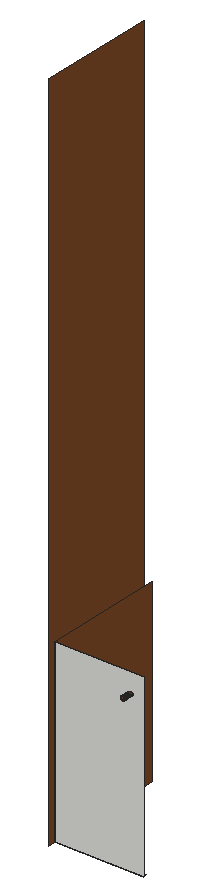
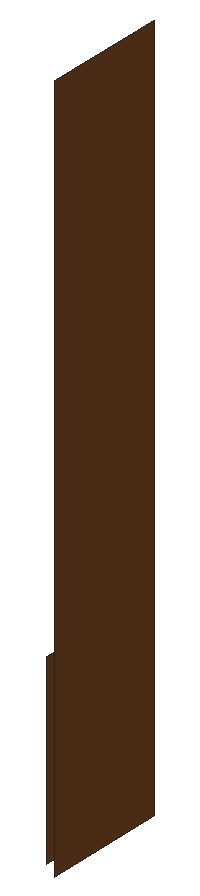
# SketchUp Ruby script. Lengths in inches.
U = 1.inch
M = Sketchup.active_model
def pt(a) = Geom::Point3d.new(a.map { |v| v * U })
def face(e, loops, mat)
  f = e.add_face(loops[0].map { |a| pt(a) })
  loops[1..].each { |l| e.add_face(l.map { |a| pt(a) }).erase! }
  f.material = f.back_material = mat if mat
  f
end
# faces: each face lists its corners as indices into pts; further lists are holes
def faces(e, pts, list, mat = nil) = list.each { |f| face(e, (f[0].is_a?(Array) ? f : [f]).map { |l| l.map { |i| pts[i] } }, mat) }
# xy, xz, yz: faces in a plane at the given z, y or x. An outline is a flat list of corners, or four numbers for a rectangle; further outlines are holes
def ring(l) = l.size == 4 ? [[l[0], l[1]], [l[2], l[1]], [l[2], l[3]], [l[0], l[3]]] : l.each_slice(2).to_a
def flat(e, list, mat, &to3) = list.each { |f| face(e, (f[0].is_a?(Array) ? f : [f]).map { |l| ring(l).map { |u, v| to3.(u, v) } }, mat) }
def xy(e, z, list, mat = nil) = flat(e, list, mat) { |x, y| [x, y, z] }
def xz(e, y, list, mat = nil) = flat(e, list, mat) { |x, z| [x, y, z] }
def yz(e, x, list, mat = nil) = flat(e, list, mat) { |y, z| [x, y, z] }
def lines(e, pts, list) = list.each { |a, b| e.add_line(pt(pts[a]), pt(pts[b])) }
# prism: a flat outline (further loops are holes) pulled along v
def prism(e, loops, v, mat = nil)
  f = face(e, loops, mat); d = Geom::Vector3d.new(v.map { |x| x * U })
  f.pushpull(f.normal.samedirection?(d) ? d.length : -d.length)
end
def box(e, o, s, mat = nil) = prism(e, [[o, [o[0] + s[0], o[1], o[2]], [o[0] + s[0], o[1] + s[1], o[2]], [o[0], o[1] + s[1], o[2]]]], [0, 0, s[2]], mat)
def at(x, y, z, deg = 0) = Geom::Transformation.translation(pt([x, y, z])) * Geom::Transformation.rotation(ORIGIN, Z_AXIS, deg.degrees)
def axes(o, x, y, z) = Geom::Transformation.new([*x, 0, *y, 0, *z, 0, *pt(o).to_a, 1])
def part(name) = M.definitions.add(name)
# library, detail: a bought-in or finely detailed component or shape, given as its bounding box
def library(name, o, s) = part(name).tap { |d| box(d.entities, o, s) }
def detail(e, o, s) = box(e.add_group.entities, o, s)
def put(e, d, t, mat = nil) = e.add_instance(d, t).tap { |i| i.material = mat if mat }
def group(e, t, mat = nil) = e.add_group.tap { |g| g.transformation = t; g.material = mat if mat }.entities
root = M.entities
M.materials.add("[Wood Veneer 01]").color = [120, 70, 37]
xy(root,1.59,[[12.383,2,30.265,2.472]],"[Wood Veneer 01]")
xz(root,0,[[27.679,33.388,27.679,33.406,27.608,33.416,27.603,33.398],[27.679,33.388,27.756,33.398,27.751,33.416,27.679,33.406],[27.603,33.398,27.608,33.416,27.541,33.444,27.532,33.428],[27.756,33.398,27.827,33.428,27.818,33.444,27.751,33.416],[27.679,33.406,27.751,33.416,27.818,33.444,27.875,33.488,27.919,33.545,27.947,33.612,27.956,33.683,27.947,33.755,27.919,33.822,27.875,33.879,27.818,33.923,27.751,33.951,27.679,33.96,27.608,33.951,27.541,33.923,27.484,33.879,27.44,33.822,27.412,33.755,27.402,33.683,27.412,33.612,27.44,33.545,27.484,33.488,27.541,33.444,27.608,33.416],
  [27.532,33.428,27.541,33.444,27.484,33.488,27.471,33.475],[27.827,33.428,27.888,33.475,27.875,33.488,27.818,33.444],[27.471,33.475,27.484,33.488,27.44,33.545,27.424,33.536],[27.888,33.475,27.935,33.536,27.919,33.545,27.875,33.488],[27.424,33.536,27.44,33.545,27.412,33.612,27.394,33.607],
  [27.935,33.536,27.964,33.607,27.947,33.612,27.919,33.545],[27.394,33.607,27.412,33.612,27.402,33.683,27.384,33.683],[27.964,33.607,27.974,33.683,27.956,33.683,27.947,33.612],[27.384,33.683,27.402,33.683,27.412,33.755,27.394,33.76],[27.956,33.683,27.974,33.683,27.964,33.76,27.947,33.755]],"[Wood Veneer 01]")
xz(root,2,[[[12.383,1.59,30.265,37.59],[27.679,33.183,27.55,33.2,27.429,33.25,27.326,33.33,27.246,33.433,27.196,33.554,27.179,33.683,27.196,33.813,27.246,33.933,27.326,34.037,27.429,34.116,27.55,34.166,27.679,34.183,27.809,34.166,27.929,34.116,28.033,34.037,28.112,33.933,28.162,33.813,28.179,33.683,28.162,33.554,28.112,33.433,28.033,33.33,27.929,33.25,27.809,33.2]]])
yz(root,10.793,[[2.472,0,26.472,138.34]],"[Wood Veneer 01]")
yz(root,12.383,[[2,1.59,2.472,37.59],[2.472,1.59,26.472,37.59]],"[Wood Veneer 01]")
p = [[27.679,0.046,33.249],[27.567,0.046,33.264],[27.564,0.055,33.254],[27.679,0.055,33.239],[27.679,0.038,33.259],[27.57,0.038,33.274],
  [27.792,0.046,33.264],[27.789,0.038,33.274],[27.794,0.055,33.254],[27.552,0.139,33.21],[27.434,0.139,33.259],[27.432,0.154,33.256],
  [27.552,0.154,33.206],[27.554,0.124,33.214],[27.436,0.124,33.262],[27.555,0.111,33.219],[27.439,0.111,33.267],[27.556,0.098,33.224],
  [27.442,0.098,33.272],[27.558,0.086,33.231],[27.445,0.086,33.277],[27.56,0.075,33.238],[27.449,0.075,33.284],[27.562,0.065,33.246],
  [27.453,0.065,33.291],[27.457,0.055,33.299],[27.679,0.139,33.193],[27.679,0.154,33.19],[27.679,0.124,33.197],[27.679,0.111,33.202],
  [27.679,0.098,33.208],[27.679,0.086,33.215],[27.679,0.075,33.222],[27.679,0.065,33.23],[27.797,0.065,33.246],[27.799,0.075,33.238],
  [27.801,0.086,33.231],[27.802,0.098,33.224],[27.804,0.111,33.219],[27.805,0.124,33.214],[27.806,0.139,33.21],[27.807,0.154,33.206],
  [27.906,0.065,33.291],[27.901,0.055,33.299],[27.91,0.075,33.284],[27.914,0.086,33.277],[27.917,0.098,33.272],[27.92,0.111,33.267],
  [27.922,0.124,33.262],[27.924,0.139,33.259],[27.926,0.154,33.256],[27.429,2,33.25],[27.55,2,33.2],[27.55,0.221,33.2],
  [27.429,0.221,33.25],[27.55,0.203,33.201],[27.43,0.203,33.251],[27.55,0.186,33.202],[27.43,0.186,33.252],[27.551,0.169,33.204],
  [27.431,0.169,33.253],[27.679,2,33.183],[27.679,0.221,33.183],[27.679,0.203,33.184],[27.679,0.186,33.185],[27.679,0.169,33.187],
  [27.808,0.169,33.204],[27.808,0.186,33.202],[27.809,0.203,33.201],[27.809,0.221,33.2],[27.809,2,33.2],[27.928,0.169,33.253],
  [27.929,0.186,33.252],[27.929,0.203,33.251],[27.929,0.221,33.25],[27.929,2,33.25],[27.462,0.046,33.307],[27.372,0.046,33.376],
  [27.365,0.055,33.369],[27.467,0.038,33.316],[27.379,0.038,33.383],[27.473,0.031,33.326],[27.387,0.031,33.391],[27.479,0.025,33.336],
  [27.396,0.025,33.4],[27.485,0.019,33.347],[27.405,0.019,33.409],[27.492,0.014,33.359],[27.414,0.014,33.418],[27.572,0.031,33.285],
  [27.576,0.025,33.296],[27.579,0.019,33.308],[27.582,0.014,33.322],[27.586,0.01,33.335],[27.499,0.01,33.371],[27.59,0.006,33.35],
  [27.507,0.006,33.384],[27.594,0.003,33.365],[27.515,0.003,33.398],[27.679,0.031,33.27],[27.679,0.025,33.282],[27.679,0.019,33.295],
  [27.679,0.014,33.309],[27.679,0.01,33.323],[27.679,0.006,33.338],[27.679,0.003,33.354],[27.769,0.006,33.35],[27.765,0.003,33.365],
  [27.773,0.01,33.335],[27.776,0.014,33.322],[27.78,0.019,33.308],[27.783,0.025,33.296],[27.786,0.031,33.285],[27.852,0.006,33.384],
  [27.844,0.003,33.398],[27.859,0.01,33.371],[27.867,0.014,33.359],[27.873,0.019,33.347],[27.88,0.025,33.336],[27.886,0.031,33.326],
  [27.891,0.038,33.316],[27.897,0.046,33.307],[27.954,0.019,33.409],[27.944,0.014,33.418],[27.963,0.025,33.4],[27.971,0.031,33.391],
  [27.979,0.038,33.383],[27.987,0.046,33.376],[27.993,0.055,33.369],[27.333,0.139,33.337],[27.255,0.139,33.438],[27.252,0.154,33.436],
  [27.33,0.154,33.334],[27.336,0.124,33.34],[27.258,0.124,33.44],[27.339,0.111,33.343],[27.263,0.111,33.443],[27.343,0.098,33.347],
  [27.268,0.098,33.446],[27.348,0.086,33.352],[27.273,0.086,33.449],[27.353,0.075,33.357],[27.359,0.065,33.363],[28,0.065,33.363],
  [28.005,0.075,33.357],[28.011,0.086,33.352],[28.015,0.098,33.347],[28.019,0.111,33.343],[28.023,0.124,33.34],[28.026,0.139,33.337],
  [28.028,0.154,33.334],[28.091,0.098,33.446],[28.085,0.086,33.449],[28.096,0.111,33.443],[28.1,0.124,33.44],[28.104,0.139,33.438],
  [28.107,0.154,33.436],[27.246,2,33.433],[27.326,2,33.33],[27.326,0.221,33.33],[27.246,0.221,33.433],[27.326,0.203,33.33],
  [27.247,0.203,33.433],[27.327,0.186,33.331],[27.248,0.186,33.434],[27.328,0.169,33.332],[27.249,0.169,33.435],[28.03,0.169,33.332],
  [28.032,0.186,33.331],[28.033,0.203,33.33],[28.033,0.221,33.33],[28.033,2,33.33],[28.109,0.169,33.435],[28.111,0.186,33.434],
  [28.112,0.203,33.433],[28.112,0.221,33.433],[28.112,2,33.433],[27.303,0.046,33.466],[27.295,0.055,33.461],[27.312,0.038,33.471],
  [27.322,0.031,33.477],[27.332,0.025,33.483],[27.343,0.019,33.489],[27.355,0.014,33.496],[27.425,0.01,33.429],[27.367,0.01,33.503],
  [27.435,0.006,33.439],[27.38,0.006,33.511],[27.447,0.003,33.451],[27.394,0.003,33.519],[27.523,0.002,33.413],[27.458,0.002,33.462],
  [27.532,0,33.428],[27.471,0,33.475],[27.598,0.002,33.381],[27.603,0,33.398],[27.679,0.002,33.371],[27.679,0,33.388],
  [27.76,0.002,33.381],[27.756,0,33.398],[27.836,0.002,33.413],[27.827,0,33.428],[27.9,0.002,33.462],[27.888,0,33.475],
  [27.912,0.003,33.451],[27.923,0.006,33.439],[27.934,0.01,33.429],[27.978,0.006,33.511],[27.964,0.003,33.519],[27.991,0.01,33.503],
  [28.004,0.014,33.496],[28.015,0.019,33.489],[28.026,0.025,33.483],[28.037,0.031,33.477],[28.047,0.038,33.471],[28.056,0.046,33.466],
  [28.064,0.055,33.461],[27.206,0.139,33.556],[27.202,0.154,33.556],[27.21,0.124,33.558],[27.215,0.111,33.559],[27.22,0.098,33.56],
  [27.227,0.086,33.562],[27.28,0.075,33.453],[27.234,0.075,33.564],[27.287,0.065,33.457],[28.072,0.065,33.457],[28.079,0.075,33.453],
  [28.125,0.075,33.564],[28.132,0.086,33.562],[28.138,0.098,33.56],[28.144,0.111,33.559],[28.149,0.124,33.558],[28.153,0.139,33.556],
  [28.156,0.154,33.556],[27.196,2,33.554],[27.196,0.221,33.554],[27.197,0.203,33.554],[27.198,0.186,33.554],[27.2,0.169,33.555],
  [28.159,0.169,33.555],[28.161,0.186,33.554],[28.162,0.203,33.554],[28.162,0.221,33.554],[28.162,2,33.554],[27.26,0.046,33.571],
  [27.25,0.055,33.568],[27.27,0.038,33.574],[27.281,0.031,33.576],[27.292,0.025,33.58],[27.304,0.019,33.583],[27.318,0.014,33.586],
  [27.331,0.01,33.59],[27.346,0.006,33.594],[27.361,0.003,33.598],[27.409,0.002,33.527],[27.377,0.002,33.602],[27.424,0,33.536],
  [27.394,0,33.607],[27.95,0.002,33.527],[27.935,0,33.536],[27.964,0,33.607],[27.981,0.002,33.602],[27.997,0.003,33.598],
  [28.013,0.006,33.594],[28.027,0.01,33.59],[28.041,0.014,33.586],[28.054,0.019,33.583],[28.066,0.025,33.58],[28.078,0.031,33.576],
  [28.089,0.038,33.574],[28.099,0.046,33.571],[28.108,0.055,33.568],[27.242,0.065,33.566],[28.117,0.065,33.566],[27.245,0.046,33.683],
  [27.235,0.055,33.683],[27.255,0.038,33.683],[27.266,0.031,33.683],[27.278,0.025,33.683],[27.291,0.019,33.683],[27.305,0.014,33.683],
  [27.319,0.01,33.683],[27.334,0.006,33.683],[27.35,0.003,33.683],[27.367,0.002,33.683],[27.384,0,33.683],[27.992,0.002,33.683],
  [27.974,0,33.683],[28.009,0.003,33.683],[28.024,0.006,33.683],[28.039,0.01,33.683],[28.054,0.014,33.683],[28.067,0.019,33.683],
  [28.08,0.025,33.683],[28.092,0.031,33.683],[28.103,0.038,33.683],[28.114,0.046,33.683],[28.124,0.055,33.683],[27.189,0.139,33.683],
  [27.186,0.154,33.683],[27.193,0.124,33.683],[27.198,0.111,33.683],[27.204,0.098,33.683],[27.211,0.086,33.683],[27.218,0.075,33.683],
  [27.226,0.065,33.683],[28.132,0.065,33.683],[28.141,0.075,33.683],[28.148,0.086,33.683],[28.155,0.098,33.683],[28.16,0.111,33.683],
  [28.165,0.124,33.683],[28.17,0.139,33.683],[28.173,0.154,33.683],[27.179,2,33.683],[27.179,0.221,33.683],[27.18,0.203,33.683],
  [27.181,0.186,33.683],[27.183,0.169,33.683],[28.176,0.169,33.683],[28.178,0.186,33.683],[28.179,0.203,33.683],[28.179,0.221,33.683],
  [28.179,2,33.683],[27.26,0.046,33.796],[27.25,0.055,33.798],[27.27,0.038,33.793],[27.281,0.031,33.79],[27.292,0.025,33.787],
  [27.304,0.019,33.784],[27.318,0.014,33.78],[27.331,0.01,33.777],[27.346,0.006,33.773],[27.361,0.003,33.769],[27.377,0.002,33.764],
  [27.394,0,33.76],[27.964,0,33.76],[27.981,0.002,33.764],[27.997,0.003,33.769],[28.013,0.006,33.773],[28.027,0.01,33.777],
  [28.041,0.014,33.78],[28.054,0.019,33.784],[28.066,0.025,33.787],[28.078,0.031,33.79],[28.089,0.038,33.793],[28.099,0.046,33.796],
  [28.108,0.055,33.798],[27.206,0.139,33.81],[27.202,0.154,33.811],[27.21,0.124,33.809],[27.215,0.111,33.808],[27.22,0.098,33.806],
  [27.227,0.086,33.805],[27.234,0.075,33.803],[27.242,0.065,33.801],[28.117,0.065,33.801],[28.125,0.075,33.803],[28.132,0.086,33.805],
  [28.138,0.098,33.806],[28.144,0.111,33.808],[28.149,0.124,33.809],[28.153,0.139,33.81],[28.156,0.154,33.811],[27.196,2,33.813],
  [27.196,0.221,33.813],[27.197,0.203,33.8125],[27.198,0.186,33.8125],[27.2,0.169,33.812],[28.159,0.169,33.812],[28.161,0.186,33.8125],
  [28.162,0.203,33.8125],[28.162,0.221,33.813]]
faces(root,p,[[0,1,2,3],[4,5,1,0],[0,6,7,4],[3,8,6,0],[9,10,11,12],[13,14,10,9],[15,16,14,13],[17,18,16,15],
  [19,20,18,17],[21,22,20,19],[23,24,22,21],[2,25,24,23],[26,9,12,27],[28,13,9,26],[29,15,13,28],[30,17,15,29],
  [31,19,17,30],[32,21,19,31],[33,23,21,32],[3,2,23,33],[33,34,8,3],[32,35,34,33],[31,36,35,32],[30,37,36,31],
  [29,38,37,30],[28,39,38,29],[26,40,39,28],[27,41,40,26],[34,42,43,8],[35,44,42,34],[36,45,44,35],[37,46,45,36],
  [38,47,46,37],[39,48,47,38],[40,49,48,39],[41,50,49,40],[51,52,53,54],[55,56,54,53],[57,58,56,55],[59,60,58,57],
  [12,11,60,59],[52,61,62,53],[63,55,53,62],[64,57,55,63],[65,59,57,64],[27,12,59,65],[65,66,41,27],[64,67,66,65],
  [63,68,67,64],[62,69,68,63],[61,70,69,62],[66,71,50,41],[67,72,71,66],[68,73,72,67],[69,74,73,68],[70,75,74,69],
  [76,77,78,25],[79,80,77,76],[81,82,80,79],[83,84,82,81],[85,86,84,83],[87,88,86,85],[1,76,25,2],[5,79,76,1],
  [89,81,79,5],[90,83,81,89],[91,85,83,90],[92,87,85,91],[93,94,87,92],[95,96,94,93],[97,98,96,95],[99,89,5,4],
  [100,90,89,99],[101,91,90,100],[102,92,91,101],[103,93,92,102],[104,95,93,103],[105,97,95,104],[104,106,107,105],[103,108,106,104],
  [102,109,108,103],[101,110,109,102],[100,111,110,101],[99,112,111,100],[4,7,112,99],[106,113,114,107],[108,115,113,106],[109,116,115,108],
  [110,117,116,109],[111,118,117,110],[112,119,118,111],[7,120,119,112],[6,121,120,7],[8,43,121,6],[117,122,123,116],[118,124,122,117],
  [119,125,124,118],[120,126,125,119],[121,127,126,120],[43,128,127,121],[129,130,131,132],[133,134,130,129],[135,136,134,133],[137,138,136,135],
  [139,140,138,137],[10,129,132,11],[14,133,129,10],[16,135,133,14],[18,137,135,16],[20,139,137,18],[22,141,139,20],[24,142,141,22],
  [25,78,142,24],[42,143,128,43],[44,144,143,42],[45,145,144,44],[46,146,145,45],[47,147,146,46],[48,148,147,47],[49,149,148,48],
  [50,150,149,49],[146,151,152,145],[147,153,151,146],[148,154,153,147],[149,155,154,148],[150,156,155,149],[157,158,159,160],[161,162,160,159],
  [163,164,162,161],[165,166,164,163],[132,131,166,165],[158,51,54,159],[56,161,159,54],[58,163,161,56],[60,165,163,58],[11,132,165,60],
  [71,167,150,50],[72,168,167,71],[73,169,168,72],[74,170,169,73],[75,171,170,74],[167,172,156,150],[168,173,172,167],[169,174,173,168],
  [170,175,174,169],[171,176,175,170],[77,177,178,78],[80,179,177,77],[82,180,179,80],[84,181,180,82],[86,182,181,84],[88,183,182,86],
  [184,185,183,88],[186,187,185,184],[188,189,187,186],[94,184,88,87],[96,186,184,94],[98,188,186,96],[190,191,188,98],[192,193,191,190],
  [194,190,98,97],[195,192,190,194],[196,194,97,105],[197,195,194,196],[196,198,199,197],[105,107,198,196],[198,200,201,199],[107,114,200,198],
  [200,202,203,201],[114,204,202,200],[113,205,204,114],[115,206,205,113],[116,123,206,115],[205,207,208,204],[206,209,207,205],[123,210,209,206],
  [122,211,210,123],[124,212,211,122],[125,213,212,124],[126,214,213,125],[127,215,214,126],[128,216,215,127],[130,217,218,131],[134,219,217,130],
  [136,220,219,134],[138,221,220,136],[140,222,221,138],[223,224,222,140],[141,223,140,139],[142,225,223,141],[78,178,225,142],[143,226,216,128],
  [144,227,226,143],[145,152,227,144],[228,227,152,229],[229,152,151,230],[230,151,153,231],[231,153,154,232],[232,154,155,233],[233,155,156,234],
  [235,157,160,236],[162,237,236,160],[164,238,237,162],[166,239,238,164],[131,218,239,166],[234,156,172,240],[240,172,173,241],[241,173,174,242],
  [242,174,175,243],[176,244,243,175],[177,245,246,178],[179,247,245,177],[180,248,247,179],[181,249,248,180],[182,250,249,181],[183,251,250,182],
  [185,252,251,183],[187,253,252,185],[189,254,253,187],[255,256,254,189],[257,258,256,255],[191,255,189,188],[193,257,255,191],[202,259,260,203],
  [204,208,259,202],[261,260,259,262],[262,259,208,263],[263,208,207,264],[264,207,209,265],[265,209,210,266],[266,210,211,267],[267,211,212,268],
  [268,212,213,269],[269,213,214,270],[270,214,215,271],[271,215,216,272],[225,273,224,223],[178,246,273,225],[272,216,226,274],[274,226,227,228],
  [245,275,276,246],[247,277,275,245],[248,278,277,247],[249,279,278,248],[250,280,279,249],[251,281,280,250],[252,282,281,251],[253,283,282,252],
  [254,284,283,253],[256,285,284,254],[258,286,285,256],[262,287,288,261],[263,289,287,262],[264,290,289,263],[265,291,290,264],[266,292,291,265],
  [267,293,292,266],[268,294,293,267],[269,295,294,268],[270,296,295,269],[271,297,296,270],[272,298,297,271],[217,299,300,218],[219,301,299,217],
  [220,302,301,219],[221,303,302,220],[222,304,303,221],[224,305,304,222],[273,306,305,224],[246,276,306,273],[274,307,298,272],[228,308,307,274],
  [229,309,308,228],[230,310,309,229],[231,311,310,230],[232,312,311,231],[233,313,312,232],[234,314,313,233],[315,235,236,316],[237,317,316,236],
  [238,318,317,237],[239,319,318,238],[218,300,319,239],[240,320,314,234],[241,321,320,240],[242,322,321,241],[243,323,322,242],[244,324,323,243],
  [275,325,326,276],[277,327,325,275],[278,328,327,277],[279,329,328,278],[280,330,329,279],[281,331,330,280],[282,332,331,281],[283,333,332,282],
  [284,334,333,283],[285,335,334,284],[286,336,335,285],[337,288,287,338],[338,287,289,339],[339,289,290,340],[340,290,291,341],[341,291,292,342],
  [342,292,293,343],[343,293,294,344],[344,294,295,345],[345,295,296,346],[346,296,297,347],[347,297,298,348],[299,349,350,300],[301,351,349,299],
  [302,352,351,301],[303,353,352,302],[304,354,353,303],[305,355,354,304],[306,356,355,305],[276,326,356,306],[348,298,307,357],[357,307,308,358],
  [358,308,309,359],[359,309,310,360],[360,310,311,361],[361,311,312,362],[362,312,313,363],[363,313,314,364],[365,315,316,366],[317,367,366,316],
  [318,368,367,317],[319,369,368,318],[300,350,369,319],[364,314,320,370],[370,320,321,371],[371,321,322,372],[372,322,323,373]],"[Wood Veneer 01]")
